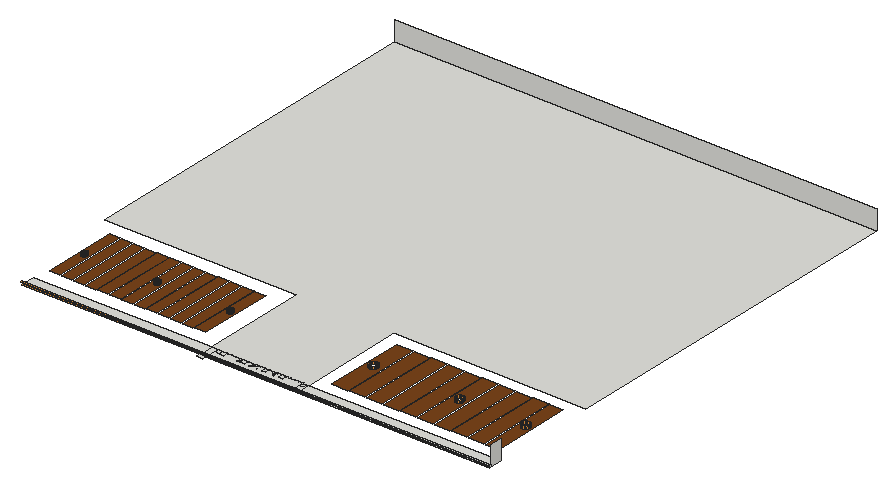
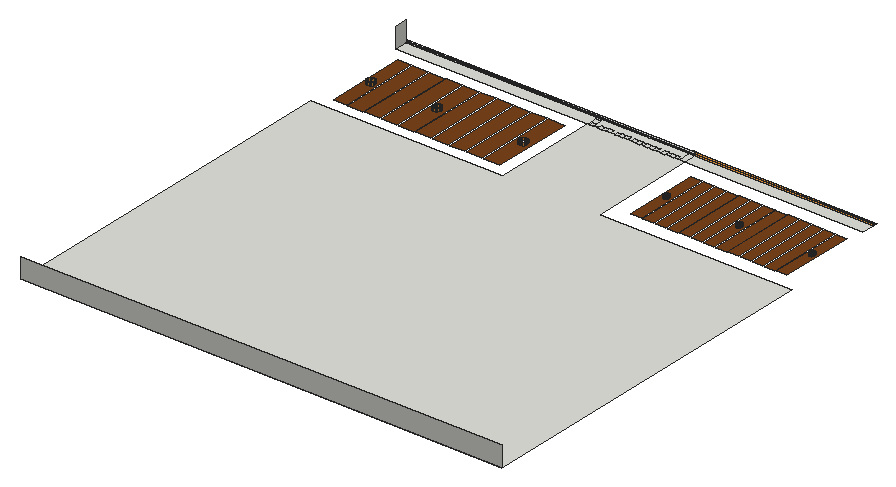
# SketchUp Ruby script. Lengths in inches.
U = 1.inch
M = Sketchup.active_model
def pt(a) = Geom::Point3d.new(a.map { |v| v * U })
def face(e, loops, mat)
  f = e.add_face(loops[0].map { |a| pt(a) })
  loops[1..].each { |l| e.add_face(l.map { |a| pt(a) }).erase! }
  f.material = f.back_material = mat if mat
  f
end
# faces: each face lists its corners as indices into pts; further lists are holes
def faces(e, pts, list, mat = nil) = list.each { |f| face(e, (f[0].is_a?(Array) ? f : [f]).map { |l| l.map { |i| pts[i] } }, mat) }
# xy, xz, yz: faces in a plane at the given z, y or x. An outline is a flat list of corners, or four numbers for a rectangle; further outlines are holes
def ring(l) = l.size == 4 ? [[l[0], l[1]], [l[2], l[1]], [l[2], l[3]], [l[0], l[3]]] : l.each_slice(2).to_a
def flat(e, list, mat, &to3) = list.each { |f| face(e, (f[0].is_a?(Array) ? f : [f]).map { |l| ring(l).map { |u, v| to3.(u, v) } }, mat) }
def xy(e, z, list, mat = nil) = flat(e, list, mat) { |x, y| [x, y, z] }
def xz(e, y, list, mat = nil) = flat(e, list, mat) { |x, z| [x, y, z] }
def yz(e, x, list, mat = nil) = flat(e, list, mat) { |y, z| [x, y, z] }
def lines(e, pts, list) = list.each { |a, b| e.add_line(pt(pts[a]), pt(pts[b])) }
# prism: a flat outline (further loops are holes) pulled along v
def prism(e, loops, v, mat = nil)
  f = face(e, loops, mat); d = Geom::Vector3d.new(v.map { |x| x * U })
  f.pushpull(f.normal.samedirection?(d) ? d.length : -d.length)
end
def box(e, o, s, mat = nil) = prism(e, [[o, [o[0] + s[0], o[1], o[2]], [o[0] + s[0], o[1] + s[1], o[2]], [o[0], o[1] + s[1], o[2]]]], [0, 0, s[2]], mat)
def at(x, y, z, deg = 0) = Geom::Transformation.translation(pt([x, y, z])) * Geom::Transformation.rotation(ORIGIN, Z_AXIS, deg.degrees)
def axes(o, x, y, z) = Geom::Transformation.new([*x, 0, *y, 0, *z, 0, *pt(o).to_a, 1])
def part(name) = M.definitions.add(name)
# library, detail: a bought-in or finely detailed component or shape, given as its bounding box
def library(name, o, s) = part(name).tap { |d| box(d.entities, o, s) }
def detail(e, o, s) = box(e.add_group.entities, o, s)
def put(e, d, t, mat = nil) = e.add_instance(d, t).tap { |i| i.material = mat if mat }
def group(e, t, mat = nil) = e.add_group.tap { |g| g.transformation = t; g.material = mat if mat }.entities
root = M.entities
M.materials.add("Generic\#1").color = [121, 68, 27]
M.materials.add("Generic\#2").color = [245, 199, 133]
M.materials.add("Generic\#4").color = [232, 149, 60]
xy(root,542.625,[[204.09,35.5625,210.09,39.5],[204.09,39.5,210.09,41],[210.09,39.5,507.875,41],[17.125,41,204.09,54.5625],[204.09,41,210.09,54.5625],
  [210.09,41,210.09,54.5625,211.72,54.5625,211.72,49.875,215.72,49.875,215.72,54.5625,300.09,54.5625,300.09,43.625,306.09,43.625,306.09,54.5625,507.875,54.5625,507.875,41],[300.09,43.625,300.09,54.5625,300.47,54.5625,300.47,49.875,304.47,49.875,304.47,54.5625,306.09,54.5625,306.09,43.625],[211.72,49.875,215.72,54.5625],[211.72,49.875,215.72,54.5625],[216.16,49.875,220.16,54.5625],
  [220.59,49.875,224.59,54.5625],[225.03,49.875,229.03,54.5625],[229.47,49.875,233.47,54.5625],[233.91,49.875,237.91,54.5625],[238.34,49.875,242.34,54.5625],
  [242.78,49.875,246.78,54.5625],[247.22,49.875,251.22,54.5625],[251.66,49.875,255.66,54.5625],[256.09,49.875,260.09,54.5625],[260.53,49.875,264.53,54.5625],
  [264.97,49.875,268.97,54.5625],[269.41,49.875,273.41,54.5625],[273.84,49.875,277.84,54.5625],[278.28,49.875,282.28,54.5625],[282.72,49.875,286.72,54.5625],
  [287.16,49.875,291.16,54.5625],[291.59,49.875,295.59,54.5625],[296.03,49.875,300.03,54.5625],[300.47,49.875,304.47,54.5625],[300.47,49.875,304.47,54.5625],
  [204.09,54.5625,204.09,166.1875,2.3125,166.1875,2.3125,546.8125,507.875,546.8125,507.875,166.1875,306.09,166.1875,306.09,54.5625]])
xy(root,542.625,[[[319.4375,67.9,336.375,152.84],[327.25,107.79,328.38,107.79,329.47,108.08,330.44,108.64,331.24,109.4375,331.8,110.41,332.1,111.5,332.1,112.625,331.81,113.71,331.25,114.6875,330.45,115.48,329.48,116.05,328.39,116.34,327.26,116.34,326.18,116.05,325.2,115.49,324.4,114.7,323.84,113.72,323.55,112.64,323.54,111.51,323.83,110.42,324.4,109.45,325.19,108.65,326.17,108.08]],[338.375,67.9,354.1875,152.84],[356.1875,67.9,372,152.84],[374,67.9,389.8125,152.84],[391.8125,67.9,407.625,152.84],
  [[409.625,67.9,425.4375,152.84],[417.81,107.79,418.94,107.79,420.03,108.08,421,108.64,421.8,109.4375,422.37,110.41,422.66,111.5,422.66,112.625,422.37,113.71,421.81,114.6875,421.01,115.48,420.04,116.05,418.95,116.34,417.83,116.34,416.74,116.05,415.76,115.49,414.97,114.7,414.4,113.72,414.11,112.64,414.11,111.51,414.4,110.42,414.96,109.45,415.75,108.65,416.73,108.08]],[427.4375,67.9,443.25,152.84],[445.25,67.9,461.0625,152.84],[463.0625,67.9,478.875,152.84],[[480.875,67.9,494.53,152.84],[487.25,107.79,488.38,107.79,489.47,108.08,490.44,108.64,491.24,109.4375,491.8,110.41,492.1,111.5,492.1,112.625,491.81,113.71,491.25,114.6875,490.45,115.48,489.48,116.05,488.39,116.34,487.26,116.34,486.18,116.05,485.2,115.49,484.4,114.7,483.84,113.72,483.55,112.64,483.54,111.51,483.83,110.42,484.4,109.45,485.19,108.65,486.17,108.08]],
  [[20.65,70.9,31.4,149.85],[26.07,107.35,26.8125,107.42,27.52,107.67,28.13,108.1,28.62,108.68,28.9375,109.36,29.07,110.1,29,110.84,28.75,111.55,28.32,112.16,27.75,112.65,27.07,112.97,26.33,113.1,25.58,113.03,24.875,112.78,24.26,112.35,23.77,111.78,23.46,111.1,23.32,110.36,23.39,109.61,23.64,108.9,24.07,108.29,24.65,107.8,25.33,107.49]],[33.4,70.9,44.15,149.85],[46.15,70.9,56.9,149.85],[58.9,70.9,69.65,149.85],[71.65,70.9,82.4,149.85],
  [84.4,70.9,95.15,149.85],[[97.15,70.9,107.9,149.85],[102.38,107.35,103.125,107.42,103.83,107.67,104.45,108.1,104.93,108.68,105.25,109.36,105.38,110.1,105.32,110.84,105.0625,111.55,104.63,112.16,104.06,112.65,103.38,112.97,102.64,113.1,101.89,113.03,101.1875,112.78,100.57,112.35,100.09,111.78,99.77,111.1,99.64,110.36,99.7,109.61,99.96,108.9,100.39,108.29,100.96,107.8,101.64,107.49]],[109.9,70.9,120.65,149.85],[122.65,70.9,133.4,149.85],[135.4,70.9,146.15,149.85],
  [148.15,70.9,158.9,149.85],[160.9,70.9,171.65,149.85],[[173.65,70.9,184.4,149.85],[179.07,107.35,179.8125,107.42,180.52,107.67,181.13,108.1,181.62,108.68,181.9375,109.36,182.07,110.1,182,110.84,181.75,111.55,181.32,112.16,180.75,112.65,180.07,112.97,179.33,113.1,178.58,113.03,177.875,112.78,177.26,112.35,176.77,111.78,176.46,111.1,176.32,110.36,176.39,109.61,176.64,108.9,177.07,108.29,177.65,107.8,178.33,107.49]]],"Generic\#1")
xy(root,542.625,[[17.125,39.5,204.09,41]],"Generic\#4")
xy(root,544.65,[[204.09,39.5,507.875,41]])
xy(root,544.65,[[15.3125,39.5,204.09,41]],"Generic\#4")
xz(root,107.79,[[327.25,542.625,328.38,545.1875],[417.81,542.625,418.94,545.1875],[487.25,542.625,488.38,545.1875]],"Generic\#4")
xz(root,116.34,[[327.26,542.625,328.39,545.1875],[417.83,542.625,418.95,545.1875],[487.26,542.625,488.39,545.1875]],"Generic\#4")
xz(root,546.8125,[[2.3125,542.625,507.875,563.5]])
yz(root,332.1,[[111.5,542.625,112.625,545.1875]],"Generic\#4")
yz(root,414.11,[[111.51,542.625,112.64,545.1875]],"Generic\#4")
yz(root,422.66,[[111.5,542.625,112.625,545.1875]],"Generic\#4")
yz(root,492.1,[[111.5,542.625,112.625,545.1875]],"Generic\#4")
yz(root,507.875,[[39.5,542.625,41,544.65],[41,542.625,54.5625,563.5]])
p = [[26.07,107.35,542.625],[25.33,107.49,542.625],[25.33,107.49,545.1875],[26.07,107.35,545.1875],[26.8125,107.42,542.625],[26.8125,107.42,545.1875],
  [27.52,107.67,542.625],[27.52,107.67,545.1875],[102.38,107.35,542.625],[101.64,107.49,542.625],[101.64,107.49,545.1875],[102.38,107.35,545.1875],
  [103.125,107.42,542.625],[103.125,107.42,545.1875],[103.83,107.67,542.625],[103.83,107.67,545.1875],[179.07,107.35,542.625],[178.33,107.49,542.625],
  [178.33,107.49,545.1875],[179.07,107.35,545.1875],[179.8125,107.42,542.625],[179.8125,107.42,545.1875],[180.52,107.67,542.625],[180.52,107.67,545.1875],
  [24.65,107.8,542.625],[24.65,107.8,545.1875],[100.96,107.8,542.625],[100.96,107.8,545.1875],[177.65,107.8,542.625],[177.65,107.8,545.1875],
  [28.13,108.1,542.625],[28.13,108.1,545.1875],[104.45,108.1,542.625],[104.45,108.1,545.1875],[181.13,108.1,542.625],[181.13,108.1,545.1875],
  [24.07,108.29,542.625],[24.07,108.29,545.1875],[100.39,108.29,542.625],[100.39,108.29,545.1875],[177.07,108.29,542.625],[177.07,108.29,545.1875],
  [327.25,107.79,542.625],[326.17,108.08,542.625],[326.17,108.08,545.1875],[327.25,107.79,545.1875],[329.47,108.08,542.625],[328.38,107.79,542.625],
  [328.38,107.79,545.1875],[329.47,108.08,545.1875],[417.81,107.79,542.625],[416.73,108.08,542.625],[416.73,108.08,545.1875],[417.81,107.79,545.1875],
  [420.03,108.08,542.625],[418.94,107.79,542.625],[418.94,107.79,545.1875],[420.03,108.08,545.1875],[487.25,107.79,542.625],[486.17,108.08,542.625],
  [486.17,108.08,545.1875],[487.25,107.79,545.1875],[489.47,108.08,542.625],[488.38,107.79,542.625],[488.38,107.79,545.1875],[489.47,108.08,545.1875],
  [28.62,108.68,542.625],[28.62,108.68,545.1875],[104.93,108.68,542.625],[104.93,108.68,545.1875],[181.62,108.68,542.625],[181.62,108.68,545.1875],
  [325.19,108.65,542.625],[325.19,108.65,545.1875],[330.44,108.64,542.625],[330.44,108.64,545.1875],[415.75,108.65,542.625],[415.75,108.65,545.1875],
  [421,108.64,542.625],[421,108.64,545.1875],[485.19,108.65,542.625],[485.19,108.65,545.1875],[490.44,108.64,542.625],[490.44,108.64,545.1875],
  [23.64,108.9,542.625],[23.64,108.9,545.1875],[99.96,108.9,542.625],[99.96,108.9,545.1875],[176.64,108.9,542.625],[176.64,108.9,545.1875],
  [324.4,109.45,542.625],[324.4,109.45,545.1875],[331.24,109.4375,542.625],[331.24,109.4375,545.1875],[414.96,109.45,542.625],[414.96,109.45,545.1875],
  [421.8,109.4375,542.625],[421.8,109.4375,545.1875],[484.4,109.45,542.625],[484.4,109.45,545.1875],[491.24,109.4375,542.625],[491.24,109.4375,545.1875],
  [28.9375,109.36,542.625],[28.9375,109.36,545.1875],[105.25,109.36,542.625],[105.25,109.36,545.1875],[181.9375,109.36,542.625],[181.9375,109.36,545.1875],
  [23.39,109.61,542.625],[23.39,109.61,545.1875],[99.7,109.61,542.625],[99.7,109.61,545.1875],[176.39,109.61,542.625],[176.39,109.61,545.1875],
  [29.07,110.1,542.625],[29.07,110.1,545.1875],[105.38,110.1,542.625],[105.38,110.1,545.1875],[182.07,110.1,542.625],[182.07,110.1,545.1875],
  [323.83,110.42,542.625],[323.83,110.42,545.1875],[331.8,110.41,542.625],[331.8,110.41,545.1875],[414.4,110.42,542.625],[414.4,110.42,545.1875],
  [422.37,110.41,542.625],[422.37,110.41,545.1875],[483.83,110.42,542.625],[483.83,110.42,545.1875],[491.8,110.41,542.625],[491.8,110.41,545.1875],
  [23.32,110.36,542.625],[23.32,110.36,545.1875],[99.64,110.36,542.625],[99.64,110.36,545.1875],[176.32,110.36,542.625],[176.32,110.36,545.1875],
  [29,110.84,542.625],[29,110.84,545.1875],[105.32,110.84,542.625],[105.32,110.84,545.1875],[182,110.84,542.625],[182,110.84,545.1875],
  [23.46,111.1,542.625],[23.46,111.1,545.1875],[99.77,111.1,542.625],[99.77,111.1,545.1875],[176.46,111.1,542.625],[176.46,111.1,545.1875],
  [323.54,111.51,542.625],[323.54,111.51,545.1875],[332.1,111.5,542.625],[332.1,111.5,545.1875],[414.11,111.51,542.625],[414.11,111.51,545.1875],
  [422.66,111.5,542.625],[422.66,111.5,545.1875],[483.54,111.51,542.625],[483.54,111.51,545.1875],[492.1,111.5,542.625],[492.1,111.5,545.1875],
  [28.75,111.55,542.625],[28.75,111.55,545.1875],[105.0625,111.55,542.625],[105.0625,111.55,545.1875],[181.75,111.55,542.625],[181.75,111.55,545.1875],
  [23.77,111.78,542.625],[23.77,111.78,545.1875],[100.09,111.78,542.625],[100.09,111.78,545.1875],[176.77,111.78,542.625],[176.77,111.78,545.1875],
  [28.32,112.16,542.625],[28.32,112.16,545.1875],[104.63,112.16,542.625],[104.63,112.16,545.1875],[181.32,112.16,542.625],[181.32,112.16,545.1875],
  [323.55,112.64,542.625],[323.55,112.64,545.1875],[483.55,112.64,542.625],[483.55,112.64,545.1875],[24.26,112.35,542.625],[24.26,112.35,545.1875],
  [100.57,112.35,542.625],[100.57,112.35,545.1875],[177.26,112.35,542.625],[177.26,112.35,545.1875],[27.75,112.65,542.625],[27.75,112.65,545.1875],
  [104.06,112.65,542.625],[104.06,112.65,545.1875],[180.75,112.65,542.625],[180.75,112.65,545.1875],[24.875,112.78,542.625],[24.875,112.78,545.1875],
  [101.1875,112.78,542.625],[101.1875,112.78,545.1875],[177.875,112.78,542.625],[177.875,112.78,545.1875],[27.07,112.97,542.625],[27.07,112.97,545.1875],
  [103.38,112.97,542.625],[103.38,112.97,545.1875],[180.07,112.97,542.625],[180.07,112.97,545.1875],[323.84,113.72,542.625],[323.84,113.72,545.1875],
  [331.81,113.71,542.625],[332.1,112.625,542.625],[332.1,112.625,545.1875],[331.81,113.71,545.1875],[414.11,112.64,542.625],[414.4,113.72,542.625],
  [414.4,113.72,545.1875],[414.11,112.64,545.1875],[422.37,113.71,542.625],[422.66,112.625,542.625],[422.66,112.625,545.1875],[422.37,113.71,545.1875],
  [483.84,113.72,542.625],[483.84,113.72,545.1875],[491.81,113.71,542.625],[492.1,112.625,542.625],[492.1,112.625,545.1875],[491.81,113.71,545.1875],
  [25.58,113.03,542.625],[25.58,113.03,545.1875],[101.89,113.03,542.625],[101.89,113.03,545.1875],[178.58,113.03,542.625],[178.58,113.03,545.1875],
  [26.33,113.1,542.625],[26.33,113.1,545.1875],[102.64,113.1,542.625],[102.64,113.1,545.1875],[179.33,113.1,542.625],[179.33,113.1,545.1875],
  [324.4,114.7,542.625],[324.4,114.7,545.1875],[331.25,114.6875,542.625],[331.25,114.6875,545.1875],[414.97,114.7,542.625],[414.97,114.7,545.1875],
  [421.81,114.6875,542.625],[421.81,114.6875,545.1875],[484.4,114.7,542.625],[484.4,114.7,545.1875],[491.25,114.6875,542.625],[491.25,114.6875,545.1875],
  [325.2,115.49,542.625],[325.2,115.49,545.1875],[330.45,115.48,542.625],[330.45,115.48,545.1875],[415.76,115.49,542.625],[415.76,115.49,545.1875],
  [421.01,115.48,542.625],[421.01,115.48,545.1875],[485.2,115.49,542.625],[485.2,115.49,545.1875],[490.45,115.48,542.625],[490.45,115.48,545.1875],
  [326.18,116.05,542.625],[326.18,116.05,545.1875],[329.48,116.05,542.625],[329.48,116.05,545.1875],[416.74,116.05,542.625],[416.74,116.05,545.1875],
  [420.04,116.05,542.625],[420.04,116.05,545.1875],[486.18,116.05,542.625],[486.18,116.05,545.1875],[489.48,116.05,542.625],[489.48,116.05,545.1875],
  [328.39,116.34,542.625],[328.39,116.34,545.1875],[418.95,116.34,542.625],[418.95,116.34,545.1875],[488.39,116.34,542.625],[488.39,116.34,545.1875],
  [327.26,116.34,542.625],[327.26,116.34,545.1875],[417.83,116.34,542.625],[417.83,116.34,545.1875],[487.26,116.34,542.625],[487.26,116.34,545.1875]]
faces(root,p,[[0,1,2,3],[4,0,3,5],[6,4,5,7],[8,9,10,11],[12,8,11,13],[14,12,13,15],[16,17,18,19],[20,16,19,21],
  [22,20,21,23],[1,24,25,2],[9,26,27,10],[17,28,29,18],[30,6,7,31],[32,14,15,33],[34,22,23,35],[24,36,37,25],
  [26,38,39,27],[28,40,41,29],[66,30,31,67],[68,32,33,69],[70,34,35,71],[36,84,85,37],[38,86,87,39],[40,88,89,41],
  [102,66,67,103],[104,68,69,105],[106,70,71,107],[84,108,109,85],[86,110,111,87],[88,112,113,89],[114,102,103,115],[116,104,105,117],
  [118,106,107,119],[108,132,133,109],[110,134,135,111],[112,136,137,113],[138,114,115,139],[140,116,117,141],[142,118,119,143],[132,144,145,133],
  [134,146,147,135],[136,148,149,137],[162,138,139,163],[164,140,141,165],[166,142,143,167],[144,168,169,145],[146,170,171,147],[148,172,173,149],
  [174,162,163,175],[176,164,165,177],[178,166,167,179],[168,184,185,169],[170,186,187,171],[172,188,189,173],[190,174,175,191],[192,176,177,193],
  [194,178,179,195],[184,196,197,185],[186,198,199,187],[188,200,201,189],[202,190,191,203],[204,192,193,205],[206,194,195,207],[196,228,229,197],
  [198,230,231,199],[200,232,233,201],[228,234,235,229],[234,202,203,235],[230,236,237,231],[236,204,205,237],[232,238,239,233],[238,206,207,239]],"Generic\#2")
faces(root,p,[[42,43,44,45],[46,47,48,49],[50,51,52,53],[54,55,56,57],[58,59,60,61],[62,63,64,65],[43,72,73,44],[74,46,49,75],
  [51,76,77,52],[78,54,57,79],[59,80,81,60],[82,62,65,83],[72,90,91,73],[92,74,75,93],[76,94,95,77],[96,78,79,97],
  [80,98,99,81],[100,82,83,101],[90,120,121,91],[122,92,93,123],[94,124,125,95],[126,96,97,127],[98,128,129,99],[130,100,101,131],
  [120,150,151,121],[152,122,123,153],[124,154,155,125],[156,126,127,157],[128,158,159,129],[160,130,131,161],[150,180,181,151],[158,182,183,159],
  [180,208,209,181],[210,211,212,213],[214,215,216,217],[218,219,220,221],[182,222,223,183],[224,225,226,227],[208,240,241,209],[242,210,213,243],
  [215,244,245,216],[246,218,221,247],[222,248,249,223],[250,224,227,251],[240,252,253,241],[254,242,243,255],[244,256,257,245],[258,246,247,259],
  [248,260,261,249],[262,250,251,263],[252,264,265,253],[266,254,255,267],[256,268,269,257],[270,258,259,271],[260,272,273,261],[274,262,263,275],
  [276,266,267,277],[278,270,271,279],[280,274,275,281],[264,282,283,265],[268,284,285,269],[272,286,287,273]],"Generic\#4")
